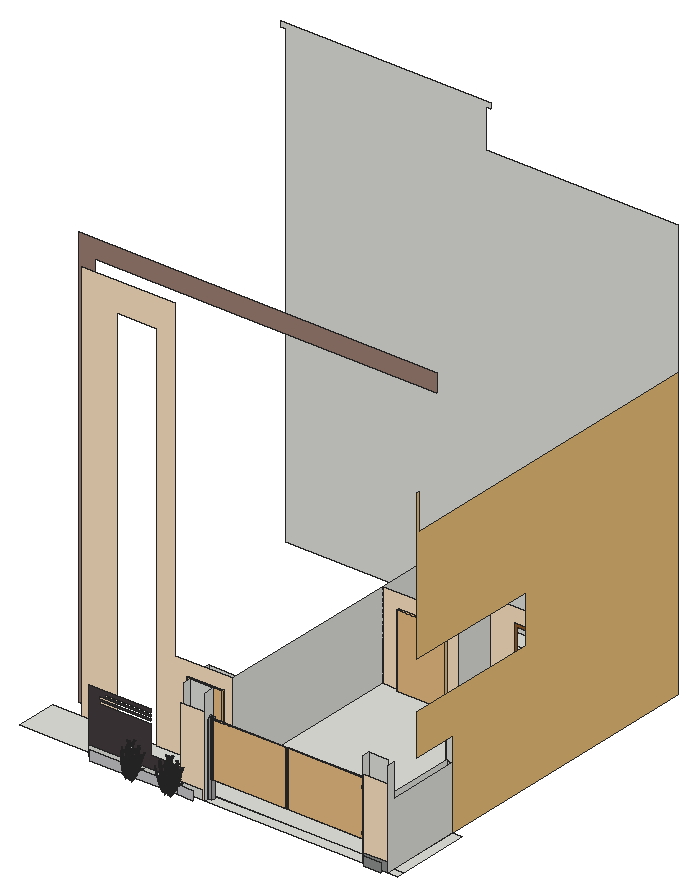
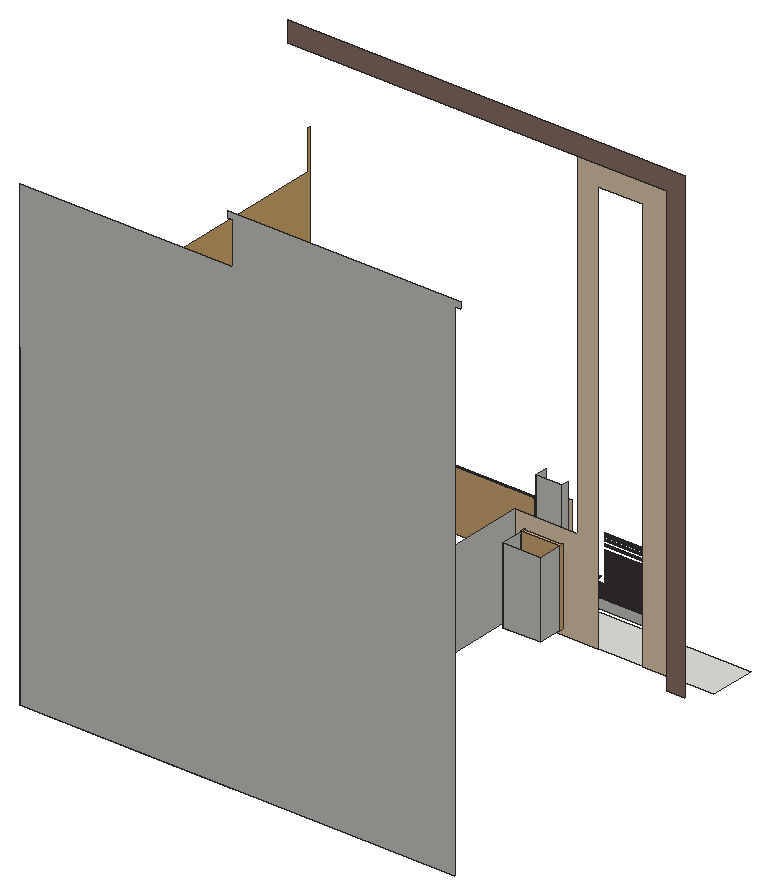
# SketchUp Ruby script. Lengths in inches.
U = 1.inch
M = Sketchup.active_model
def pt(a) = Geom::Point3d.new(a.map { |v| v * U })
def face(e, loops, mat)
  f = e.add_face(loops[0].map { |a| pt(a) })
  loops[1..].each { |l| e.add_face(l.map { |a| pt(a) }).erase! }
  f.material = f.back_material = mat if mat
  f
end
# faces: each face lists its corners as indices into pts; further lists are holes
def faces(e, pts, list, mat = nil) = list.each { |f| face(e, (f[0].is_a?(Array) ? f : [f]).map { |l| l.map { |i| pts[i] } }, mat) }
# xy, xz, yz: faces in a plane at the given z, y or x. An outline is a flat list of corners, or four numbers for a rectangle; further outlines are holes
def ring(l) = l.size == 4 ? [[l[0], l[1]], [l[2], l[1]], [l[2], l[3]], [l[0], l[3]]] : l.each_slice(2).to_a
def flat(e, list, mat, &to3) = list.each { |f| face(e, (f[0].is_a?(Array) ? f : [f]).map { |l| ring(l).map { |u, v| to3.(u, v) } }, mat) }
def xy(e, z, list, mat = nil) = flat(e, list, mat) { |x, y| [x, y, z] }
def xz(e, y, list, mat = nil) = flat(e, list, mat) { |x, z| [x, y, z] }
def yz(e, x, list, mat = nil) = flat(e, list, mat) { |y, z| [x, y, z] }
def lines(e, pts, list) = list.each { |a, b| e.add_line(pt(pts[a]), pt(pts[b])) }
# prism: a flat outline (further loops are holes) pulled along v
def prism(e, loops, v, mat = nil)
  f = face(e, loops, mat); d = Geom::Vector3d.new(v.map { |x| x * U })
  f.pushpull(f.normal.samedirection?(d) ? d.length : -d.length)
end
def box(e, o, s, mat = nil) = prism(e, [[o, [o[0] + s[0], o[1], o[2]], [o[0] + s[0], o[1] + s[1], o[2]], [o[0], o[1] + s[1], o[2]]]], [0, 0, s[2]], mat)
def at(x, y, z, deg = 0) = Geom::Transformation.translation(pt([x, y, z])) * Geom::Transformation.rotation(ORIGIN, Z_AXIS, deg.degrees)
def axes(o, x, y, z) = Geom::Transformation.new([*x, 0, *y, 0, *z, 0, *pt(o).to_a, 1])
def part(name) = M.definitions.add(name)
# library, detail: a bought-in or finely detailed component or shape, given as its bounding box
def library(name, o, s) = part(name).tap { |d| box(d.entities, o, s) }
def detail(e, o, s) = box(e.add_group.entities, o, s)
def put(e, d, t, mat = nil) = e.add_instance(d, t).tap { |i| i.material = mat if mat }
def group(e, t, mat = nil) = e.add_group.tap { |g| g.transformation = t; g.material = mat if mat }.entities
root = M.entities
M.materials.add("Niraj_Skin").color = [158, 128, 115]
M.materials.add("[0012_Bisque]").color = [255, 228, 196]
M.materials.add("[Asphalt New]").color = [67, 60, 62]
M.materials.add("[Blacktop Old 02]").color = [143, 145, 145]
M.materials.add("[Color_003]").color = [170, 170, 170]
M.materials.add("[Metal_Corrogated_Shiny]").color = [193, 193, 193]
M.materials.add("[Polished Concrete New]").color = [200, 200, 203]
M.materials.add("[Wood Floor Parquet]").color = [145, 89, 39]
M.materials.add("[Wood OSB]").color = [240, 195, 122]
M.materials.add("[Wood Veneer 02]").color = [190, 128, 91]
c1 = part("fur_instance\#8")
p = [[-0.25,1.49,0.03],[0.25,-1.49,-0.03],[0.44,-1.47,1.51],[-0.05,1.47,1.57],[0.65,-1.44,3.05],[0.16,1.45,3.11],
  [0.86,-1.42,4.59],[0.38,1.44,4.65],[1.1,-1.39,6.13],[0.62,1.43,6.18],[1.34,-1.35,7.66],[0.875,1.42,7.72],
  [1.6,-1.32,9.19],[1.14,1.41,9.25],[1.88,-1.28,10.72],[1.43,1.41,10.78],[2.18,-1.24,12.25],[1.73,1.41,12.3],
  [2.49,-1.19,13.77],[2.05,1.41,13.82],[2.83,-1.15,15.29],[2.4,1.41,15.34],[3.18,-1.09,16.8],[2.76,1.42,16.85],
  [3.56,-1.03,18.31],[3.14,1.43,18.35],[3.96,-0.97,19.81],[3.55,1.44,19.85],[4.38,-0.91,21.3],[3.99,1.46,21.35],
  [4.84,-0.83,22.78],[4.45,1.48,22.83],[5.32,-0.76,24.26],[4.93,1.51,24.31],[5.82,-0.67,25.73],[5.45,1.54,25.77],
  [6.36,-0.59,27.18],[6,1.57,27.23],[6.93,-0.49,28.625],[6.58,1.61,28.67],[7.54,-0.39,30.05],[7.19,1.66,30.1],
  [8.18,-0.28,31.47],[7.84,1.71,31.51],[8.85,-0.16,32.86],[8.53,1.77,32.9],[9.57,-0.04,34.24],[9.25,1.83,34.27],
  [10.32,0.09,35.59],[10.02,1.9,35.625],[11.12,0.23,36.92],[10.82,1.97,36.95],[11.95,0.38,38.22],[11.67,2.06,38.25],
  [12.84,0.54,39.49],[12.57,2.14,39.52],[13.76,0.71,40.73],[13.51,2.24,40.76],[14.73,0.89,41.93],[14.49,2.34,41.95],
  [15.75,1.08,43.09],[15.52,2.45,43.11],[16.82,1.28,44.2],[16.6,2.5625,44.23],[17.93,1.5,45.27],[17.73,2.68,45.29],
  [19.08,1.73,46.28],[18.9,2.81,46.3],[20.29,1.97,47.24],[20.125,2.93,47.26],[21.53,2.22,48.13],[21.39,3.0625,48.15],
  [22.82,2.5,48.96],[22.7,3.1875,48.98],[24.14,2.8125,49.72],[24.06,3.3,49.73],[25.48,3.27,50.41]]
faces(c1.entities,p,[[0,1,2,3],[3,2,4,5],[5,4,6,7],[7,6,8,9],[9,8,10,11],[11,10,12,13],[13,12,14,15],[15,14,16,17],
  [17,16,18,19],[19,18,20,21],[21,20,22,23],[23,22,24,25],[25,24,26,27],[27,26,28,29],[29,28,30,31],[31,30,32,33],
  [33,32,34,35],[35,34,36,37],[37,36,38,39],[39,38,40,41],[41,40,42,43],[43,42,44,45],[45,44,46,47],[47,46,48,49],
  [49,48,50,51],[51,50,52,53],[53,52,54,55],[55,54,56,57],[57,56,58,59],[59,58,60,61],[61,60,62,63],[63,62,64,65],
  [65,64,66,67],[67,66,68,69],[69,68,70,71],[71,70,72,73],[73,72,74,75],[75,74,76]])
c2 = library("tabla profil",[0,0,0],[95.67,0.85,78.74])
c3 = part("stilp")
box(c3.entities,[0,0,0],[4.72,4.41,106.3])
c4 = part("balama mama")
detail(c4.entities,[0,0,0],[1.18,1.18,2.76])
c5 = part("plastina balamale")
box(c5.entities,[0,0,0],[1.57,0.16,2.76])
c6 = part("balama stilp")
put(c6.entities,c4,at(1.125,0,0))
put(c6.entities,c5,at(0,1.02,0))
c7 = part("Group\#1")
put(c7.entities,c3,at(0,1.18,0))
put(c7.entities,c6,at(3.13,0,92.38))
put(c7.entities,c6,at(3.13,0,33.33))
c8 = library("Group\#2",[0,0,0],[99.09,2.17,78.74])
c9 = part("poarta+metal+2x5m")
g1 = group(c9.entities,at(-0.02,-1.18,-19.69))
put(g1,c2,at(105.29,0.33,27.56),"[Metal_Corrogated_Shiny]")
put(g1,c2,at(6.47,0.33,27.56),"[Metal_Corrogated_Shiny]")
put(g1,c7,at(0,0,0),"[Color_003]")
put(g1,c8,at(4.26,0,27.56),"[Color_003]")
put(g1,c7,axes([207.17,0,0],[-1,0,0],[0,1,0],[0,0,1]),"[Color_003]")
put(g1,c8,axes([202.92,0,27.56],[-1,0,0],[0,1,0],[0,0,1]),"[Color_003]")
c10 = library("curtain (1)",[0,0,0],[91.86,2.24,61.53])
c11 = library("porta+de+madeira",[3.7,-4.82,1.36],[53.55,7.65,83.26])
xy(root,0,[[238.24,86.15,415.52,86.15,415.52,94.44,410.77,94.44,410.77,98.26,238.24,98.26],[415.52,86.15,442.8125,86.15,442.8125,176.35,436.76,176.35,436.76,94.44,415.52,94.44],[442.8125,86.15,453.6875,94.44],[[28.64,90.32,211.95,90.32,211.95,98.26,410.77,98.26,410.77,94.44,436.76,94.44,436.76,176.35,435.86,176.35,435.86,471.23,394.67,471.23,394.67,390.22,313.66,390.22,313.66,346.4375,228.75,346.4375,228.75,136.77,28.64,136.77],[415.79,368,430.67,395.12],[418.11,240,430.67,264.5],[417.11,299.56,430.67,322]],[442.8125,94.44,443,176.35],
  [443,94.44,453.6875,176.35],[435.86,176.35,443,176.35,443,490.875,313.66,490.875,313.66,471.23,435.86,471.23],[418.11,240,430.67,242.37],[418.11,242.37,430.67,264.5],[228.75,346.4375,313.66,471.23],
  [228.75,471.23,313.66,490.875]])
xy(root,5.34,[[181.07,136.77,218.95,164.02]])
xz(root,79.88,[[115.35,0,211.95,10.375],[211.95,0,230.42,10.375]],"[Polished Concrete New]")
xz(root,82.15,[[419.51,0,438.8125,10.375]],"[Blacktop Old 02]")
xz(root,86.15,[[109.08,0,211.95,10.375],[211.95,0,236.6875,10.375]])
xz(root,86.15,[[236.6875,0,238.24,0,238.24,88.875,211.95,88.875,211.95,10.375,236.6875,10.375],[415.52,10.375,442.8125,88.875]],"[0012_Bisque]")
xz(root,86.15,[[109.08,10.375,211.95,10.375,211.95,24.89,178.5,24.89,178.5,55.78,120.75,55.78,120.75,58.72,178.5,58.72,178.5,60.82,120.5,60.82,120.5,63.13,178.5,63.13,178.5,64.89,127.31,64.89,127.31,67.33,178.5,67.33,178.5,70.5625,109.08,70.5625]],"[Asphalt New]")
xz(root,86.15,[[415.52,0,442.8125,10.375]],"[Blacktop Old 02]")
xz(root,94.44,[[415.52,0,436.76,107.1875]])
xz(root,98.26,[[211.95,0,238.24,107.1875]])
xz(root,136.77,[[[60.84,0,99.93,0,99.93,416.99,144.79,416.99,144.79,0,228.75,0,228.75,96.9375,164.91,96.9375,164.91,450.1,60.84,450.1],[181.07,5.34,218.95,81.4]]],"[0012_Bisque]")
xz(root,154.83,[[43.27,0,60.84,0,60.84,450.1,228.75,450.1,228.75,449.78,443,449.78,443,470.41,43.27,470.41]],"Niraj_Skin")
xz(root,164.02,[[181.07,5.34,218.95,81.4]])
xz(root,176.35,[[435.86,0,436.76,0,436.76,70.5625,442.8125,70.5625,442.8125,0,443,0,443,96.9375,435.86,96.9375]])
xz(root,240,[[418.11,0,430.67,78.69]],"[Wood Veneer 02]")
xz(root,264.5,[[418.11,0,418.11,78.69,419.11,78.69,419.11,100.125,430.67,100.125,430.67,0]])
xz(root,299.56,[[417.11,0,430.67,78.27]],"[Wood Veneer 02]")
xz(root,322,[[417.11,0,417.11,78.27,419.11,78.27,419.11,109.68,430.67,109.68,430.67,0]])
xz(root,346.4375,[[247.19,0,293.21,81.21]])
xz(root,346.4375,[[228.75,0,247.19,0,247.19,81.21,293.21,81.21,293.21,0,313.66,0,313.66,96.9375,228.75,96.9375]],"[0012_Bisque]")
xz(root,368,[[415.79,0,430.67,78.27]],"[Wood Veneer 02]")
xz(root,390.22,[[[313.66,0,394.67,96.9375],[341.37,19.24,374.18,80.3]]],"[0012_Bisque]")
xz(root,390.22,[[[341.37,19.24,374.18,80.3],[343.67,21.55,371.875,78]]],"[Wood Floor Parquet]")
xz(root,395.12,[[415.79,0,415.79,78.27,419.11,78.27,419.11,109.68,430.67,109.68,430.67,0]])
xz(root,471.23,[[394.67,0,435.86,96.9375]],"[0012_Bisque]")
xz(root,490.875,[[5.25,0,5.25,513.13,0,513.13,0,519.625,233.81,519.625,233.81,513.13,228.75,513.13,228.75,470.41,443,470.41,443,0]])
yz(root,181.07,[[136.77,5.34,164.02,81.4]])
yz(root,211.95,[[90.32,0,98.26,107.1875]])
yz(root,218.95,[[136.77,5.34,164.02,81.4]])
yz(root,228.75,[[136.77,0,346.4375,96.9375],[346.4375,0,471.23,96.9375]])
yz(root,238.24,[[86.15,0,98.26,107.1875]])
yz(root,313.66,[[346.4375,0,390.22,96.9375]])
yz(root,394.67,[[390.22,0,471.23,96.9375]])
yz(root,415.52,[[86.15,0,94.44,107.1875]])
yz(root,415.79,[[368,0,395.12,78.27]],"[Wood Veneer 02]")
yz(root,417.11,[[299.56,0,322,78.27]],"[Wood Veneer 02]")
yz(root,418.11,[[240,0,264.5,78.69]],"[Wood Veneer 02]")
yz(root,430.67,[[240,0,242.37,0,242.37,78.73,242.25,78.69,240,78.69],[242.37,0,264.5,0,264.5,84.8125,242.37,78.73],[299.56,0,322,0,322,80.77,302,78.27,299.56,78.27],[368,0,395.12,0,395.12,109.68,372.37,109.68,372.37,78.27,368,78.27]])
yz(root,435.86,[[176.35,0,471.23,96.9375]])
yz(root,436.76,[[94.44,0,176.35,70.5625]])
yz(root,442.8125,[[86.15,0,176.35,0,176.35,70.5625,94.44,70.5625,94.44,107.1875,86.15,107.1875]])
yz(root,443,[[176.35,0,490.875,0,490.875,322.1875,129.24,322.1875,129.24,361.9375,126.77,361.9375,126.77,195.98,278.53,195.98,278.53,142.87,126.77,142.87,126.77,96.9375,176.35,96.9375]],"[Wood OSB]")
p = [[313.66,471.23,0],[313.66,471.23,96.9375],[229.47,346.4375,0],[229.47,176.35,0]]
lines(root,p,[[0,1],[2,3]])
put(root,c1,axes([206.91,69.77,2.21],[0.10395,0.11836,-0.12851],[-0.11439,0.07411,-0.26217],[-0.07351,0.08501,0.2481]))
put(root,c1,axes([201.6,71.41,5.67],[-0.08139,0.23064,-0.15312],[-0.1699,-0.05496,-0.32193],[-0.16391,-0.02606,0.43057]))
put(root,c1,axes([162.83,72.15,2.37],[0.12897,-0.08882,0.30598],[0.12311,0.13439,-0.14076],[-0.0848,0.09806,0.28618]))
put(root,c1,axes([206.14,72.15,2.37],[0.12897,-0.08882,0.30598],[0.12311,0.13439,-0.14076],[-0.0848,0.09806,0.28618]))
put(root,c1,axes([169.21,72.82,2.47],[-0.12598,-0.09298,0.35138],[0.14548,-0.16001,0.09177],[0.09178,0.08501,0.30971]))
put(root,c1,axes([212.52,72.82,2.47],[-0.12598,-0.09298,0.35138],[0.14548,-0.16001,0.09177],[0.09178,0.08501,0.30971]))
put(root,c1,axes([168.61,74.05,5.45],[0.17475,-0.1628,0.03799],[0.13362,0.1403,-0.32315],[0.08136,0.06328,0.41208]))
put(root,c1,axes([211.92,74.05,5.45],[0.17475,-0.1628,0.03799],[0.13362,0.1403,-0.32315],[0.08136,0.06328,0.41208]))
put(root,c1,axes([167.55,73.21,2.36],[-0.04728,-0.14736,0.35137],[0.1919,-0.08682,-0.02284],[0.06183,0.09936,0.30152]))
put(root,c1,axes([210.87,73.21,2.36],[-0.04728,-0.14736,0.35137],[0.1919,-0.08682,-0.02284],[0.06183,0.09936,0.30152]))
put(root,c1,axes([168.81,74.19,4.9],[-0.12567,-0.14648,0.32324],[0.17955,-0.15616,0.02426],[0.08105,0.06304,0.41053]))
put(root,c1,axes([212.12,74.19,4.9],[-0.12567,-0.14648,0.32324],[0.17955,-0.15616,0.02426],[0.08105,0.06304,0.41053]))
put(root,c1,axes([169.69,70.52,3.26],[-0.05675,0.18901,-0.12396],[-0.14509,-0.01855,0.32364],[0.12915,0.03597,0.29172]))
put(root,c1,axes([213,70.52,3.26],[-0.05675,0.18901,-0.12396],[-0.14509,-0.01855,0.32364],[0.12915,0.03597,0.29172]))
put(root,c1,axes([162.25,73.15,3.23],[0.03058,-0.16302,0.35291],[0.18885,0.05742,0.07777],[-0.09099,0.10522,0.30707]))
put(root,c1,axes([205.5625,73.15,3.23],[0.03058,-0.16302,0.35291],[0.18885,0.05742,0.07777],[-0.09099,0.10522,0.30707]))
put(root,c1,axes([166.74,72.07,10.54],[-0.19584,0.16179,-0.00169],[-0.1515,-0.17581,0.15196],[0.03573,-0.00363,0.539]))
put(root,c1,axes([210.06,72.07,10.54],[-0.19584,0.16179,-0.00169],[-0.1515,-0.17581,0.15196],[0.03573,-0.00363,0.539]))
put(root,c1,axes([162.77,70.35,2.66],[0.12204,0.11956,-0.03437],[-0.09323,0.10261,-0.31254],[-0.10097,0.07745,0.26536]))
put(root,c1,axes([206.08,70.35,2.66],[0.12204,0.11956,-0.03437],[-0.09323,0.10261,-0.31254],[-0.10097,0.07745,0.26536]))
put(root,c1,axes([166.49,71.18,8.18],[0.03623,0.20627,-0.12936],[-0.21911,0.05324,0.03667],[0.02079,0.00357,0.48088]))
put(root,c1,axes([209.8,71.18,8.18],[0.03623,0.20627,-0.12936],[-0.21911,0.05324,0.03667],[0.02079,0.00357,0.48088]))
put(root,c1,axes([162.41,72.88,7.12],[0.2158,0.0049,0.14651],[-0.01279,0.21776,-0.18636],[-0.08047,0.03325,0.45875]))
put(root,c1,axes([205.72,72.88,7.12],[0.2158,0.0049,0.14651],[-0.01279,0.21776,-0.18636],[-0.08047,0.03325,0.45875]))
put(root,c1,axes([164.05,70.84,3.85],[-0.12886,0.11444,-0.22997],[-0.12949,-0.11784,0.12414],[-0.04678,0.07389,0.33152]))
put(root,c1,axes([207.36,70.84,3.85],[-0.12886,0.11444,-0.22997],[-0.12949,-0.11784,0.12414],[-0.04678,0.07389,0.33152]))
put(root,c1,axes([165.51,71.02,2.9375],[0.17646,0.02205,-0.09309],[-0.04854,0.13883,-0.29657],[0.00073,0.10392,0.26687]))
put(root,c1,axes([208.82,71.02,2.9375],[0.17646,0.02205,-0.09309],[-0.04854,0.13883,-0.29657],[0.00073,0.10392,0.26687]))
put(root,c1,axes([165.39,72.23,11.89],[0.11288,0.21144,-0.04258],[-0.23471,0.1258,-0.00774],[-0.00125,-0.03681,0.58142]))
put(root,c1,axes([208.7,72.23,11.89],[0.11288,0.21144,-0.04258],[-0.23471,0.1258,-0.00774],[-0.00125,-0.03681,0.58142]))
put(root,c1,axes([159.4,71.5,4.78],[0.05993,0.19956,0.02934],[-0.16765,0.09615,-0.32784],[-0.14862,0.00196,0.40149]))
put(root,c1,axes([202.71,71.5,4.78],[0.05993,0.19956,0.02934],[-0.16765,0.09615,-0.32784],[-0.14862,0.00196,0.40149]))
put(root,c1,axes([164.65,71.8,9.23],[-0.15948,0.17543,-0.11844],[-0.17074,-0.13846,0.07646],[-0.0175,0.01182,0.50519]))
put(root,c1,axes([207.96,71.8,9.23],[-0.15948,0.17543,-0.11844],[-0.17074,-0.13846,0.07646],[-0.0175,0.01182,0.50519]))
put(root,c1,axes([169.24,70.62,2.31],[-0.02741,0.17392,-0.23076],[-0.16029,0.02766,0.23757],[0.10574,0.05755,0.28081]))
put(root,c1,axes([212.55,70.62,2.31],[-0.02741,0.17392,-0.23076],[-0.16029,0.02766,0.23757],[0.10574,0.05755,0.28081]))
put(root,c1,axes([165.59,73.07,10.61],[-0.22966,0.11975,-0.02971],[-0.1055,-0.20961,0.14888],[0.00986,0.00949,0.54546]))
put(root,c1,axes([208.9,73.07,10.61],[-0.22966,0.11975,-0.02971],[-0.1055,-0.20961,0.14888],[0.00986,0.00949,0.54546]))
put(root,c1,axes([161.59,71.875,4.67],[0.149,0.11824,0.07488],[-0.1012,0.16059,-0.29075],[-0.11547,0.04466,0.37315]))
put(root,c1,axes([204.9,71.875,4.67],[0.149,0.11824,0.07488],[-0.1012,0.16059,-0.29075],[-0.11547,0.04466,0.37315]))
put(root,c1,axes([203.16,71.44,3.41],[-0.06018,0.17755,-0.31983],[-0.13865,-0.10086,-0.20049],[-0.15862,0.04585,0.31318]))
put(root,c1,axes([202.73,72.31,7.63],[-0.04995,0.23864,-0.11124],[-0.21419,-0.02204,-0.24055],[-0.12191,-0.01612,0.49664]))
put(root,c1,axes([161.89,71.77,3.15],[-0.12441,0.08913,-0.33358],[-0.11522,-0.1494,0.09624],[-0.1115,0.08552,0.29301]))
put(root,c1,axes([205.21,71.77,3.15],[-0.12441,0.08913,-0.33358],[-0.11522,-0.1494,0.09624],[-0.1115,0.08552,0.29301]))
put(root,c1,axes([169.99,72.21,7.55],[0.06433,0.21786,-0.19116],[-0.21809,0.08663,0.16557],[0.09246,-0.00116,0.48782]))
put(root,c1,axes([213.3,72.21,7.55],[0.06433,0.21786,-0.19116],[-0.21809,0.08663,0.16557],[0.09246,-0.00116,0.48782]))
put(root,c1,axes([169.59,73.11,3.22],[-0.18323,0.03397,0.2678],[0.02904,-0.19802,0.26654],[0.12063,0.06566,0.32036]))
put(root,c1,axes([212.9,73.11,3.22],[-0.18323,0.03397,0.2678],[0.02904,-0.19802,0.26654],[0.12063,0.06566,0.32036]))
put(root,c1,axes([164.06,71.89,5.04],[-0.16185,0.10098,-0.22361],[-0.11509,-0.14728,0.17524],[-0.05085,0.08033,0.3604]))
put(root,c1,axes([207.37,71.89,5.04],[-0.16185,0.10098,-0.22361],[-0.11509,-0.14728,0.17524],[-0.05085,0.08033,0.3604]))
put(root,c1,axes([166.31,71.96,6.02],[-0.1319,0.16634,-0.13442],[-0.16484,-0.10583,0.16664],[0.0172,0.04548,0.42308]))
put(root,c1,axes([209.62,71.96,6.02],[-0.1319,0.16634,-0.13442],[-0.16484,-0.10583,0.16664],[0.0172,0.04548,0.42308]))
put(root,c1,axes([166.24,72.08,3.71],[0.16157,0.07757,-0.19831],[-0.11325,0.15562,-0.18994],[0.0239,0.07619,0.35007]))
put(root,c1,axes([209.55,72.08,3.71],[0.16157,0.07757,-0.19831],[-0.11325,0.15562,-0.18994],[0.0239,0.07619,0.35007]))
put(root,c1,axes([164.1,72.54,4.23],[-0.18808,0.05687,-0.16759],[-0.06647,-0.17012,0.23097],[-0.05108,0.08069,0.36201]))
put(root,c1,axes([207.41,72.54,4.23],[-0.18808,0.05687,-0.16759],[-0.06647,-0.17012,0.23097],[-0.05108,0.08069,0.36201]))
put(root,c1,axes([165.86,71.66,2.72],[-0.17438,0.07052,-0.11324],[-0.07295,-0.12692,0.30042],[0.00076,0.10733,0.27565]))
put(root,c1,axes([209.17,71.66,2.72],[-0.17438,0.07052,-0.11324],[-0.07295,-0.12692,0.30042],[0.00076,0.10733,0.27565]))
put(root,c1,axes([159.29,73.21,2.46],[0.15352,0.06911,0.26676],[-0.03494,0.20117,-0.28887],[-0.16523,0.04776,0.32623]))
put(root,c1,axes([202.6,73.21,2.46],[0.15352,0.06911,0.26676],[-0.03494,0.20117,-0.28887],[-0.16523,0.04776,0.32623]))
put(root,c1,axes([165.14,73.51,5.21],[-0.21697,-0.00618,0.04885],[0.02773,-0.18874,0.29817],[-0.00075,0.0894,0.38532]))
put(root,c1,axes([208.45,73.51,5.21],[-0.21697,-0.00618,0.04885],[0.02773,-0.18874,0.29817],[-0.00075,0.0894,0.38532]))
put(root,c1,axes([167.67,72.27,8.23],[0.08086,0.19655,-0.23287],[-0.213,0.10459,0.05528],[0.05877,0.03065,0.4692]))
put(root,c1,axes([210.99,72.27,8.23],[0.08086,0.19655,-0.23287],[-0.213,0.10459,0.05528],[0.05877,0.03065,0.4692]))
put(root,c1,axes([160.4,72.72,7.94],[-0.0789,0.22714,-0.18379],[-0.20548,-0.06456,-0.18143],[-0.11262,0.00359,0.48952]))
put(root,c1,axes([203.71,72.72,7.94],[-0.0789,0.22714,-0.18379],[-0.20548,-0.06456,-0.18143],[-0.11262,0.00359,0.48952]))
put(root,c1,axes([166.54,74.67,4.57],[-0.18748,-0.08453,0.22152],[0.12512,-0.17975,0.22209],[0.0273,0.08703,0.39989]))
put(root,c1,axes([209.85,74.67,4.57],[-0.18748,-0.08453,0.22152],[0.12512,-0.17975,0.22209],[0.0273,0.08703,0.39989]))
put(root,c1,axes([167.96,71.4,2.67],[0.02265,0.14627,-0.32338],[-0.18321,0.06424,0.06],[0.05776,0.09281,0.28164]))
put(root,c1,axes([211.28,71.4,2.67],[0.02265,0.14627,-0.32338],[-0.18321,0.06424,0.06],[0.05776,0.09281,0.28164]))
put(root,c1,axes([168.93,72.78,9.83],[-0.06671,0.24175,-0.07521],[-0.22931,-0.04686,0.25475],[0.09711,-0.00122,0.51237]))
put(root,c1,axes([212.24,72.78,9.83],[-0.06671,0.24175,-0.07521],[-0.22931,-0.04686,0.25475],[0.09711,-0.00122,0.51237]))
put(root,c1,axes([163.52,72.73,10.38],[-0.03892,0.23857,-0.13916],[-0.24331,-0.01786,-0.06409],[-0.04532,0.0056,0.5395]))
put(root,c1,axes([206.83,72.73,10.38],[-0.03892,0.23857,-0.13916],[-0.24331,-0.01786,-0.06409],[-0.04532,0.0056,0.5395]))
put(root,c1,axes([164.64,72.03,5.51],[0.14274,0.1248,-0.18106],[-0.14873,0.12853,-0.2232],[-0.02656,0.08555,0.36591]))
put(root,c1,axes([207.96,72.03,5.51],[0.14274,0.1248,-0.18106],[-0.14873,0.12853,-0.2232],[-0.02656,0.08555,0.36591]))
put(root,c1,axes([163.76,72.71,6.8],[0.14854,0.14611,-0.10639],[-0.16099,0.14725,-0.20019],[-0.04301,0.04934,0.44533]))
put(root,c1,axes([207.07,72.71,6.8],[0.14854,0.14611,-0.10639],[-0.16099,0.14725,-0.20019],[-0.04301,0.04934,0.44533]))
put(root,c1,axes([161.33,74.08,7.08],[0.21224,0.07306,0.08848],[-0.08036,0.21667,-0.23259],[-0.08448,0.0349,0.48158]))
put(root,c1,axes([204.64,74.08,7.08],[0.21224,0.07306,0.08848],[-0.08036,0.21667,-0.23259],[-0.08448,0.0349,0.48158]))
put(root,c1,axes([161.38,73.15,2.17],[-0.14657,0.06865,-0.32949],[-0.09952,-0.16829,0.15169],[-0.11649,0.08935,0.30613]))
put(root,c1,axes([204.7,73.15,2.17],[-0.14657,0.06865,-0.32949],[-0.09952,-0.16829,0.15169],[-0.11649,0.08935,0.30613]))
put(root,c1,axes([163.86,73.3,9.57],[0.10044,0.20522,-0.10286],[-0.22219,0.11383,-0.10772],[-0.03192,0.01018,0.52996]))
put(root,c1,axes([207.18,73.3,9.57],[0.10044,0.20522,-0.10286],[-0.22219,0.11383,-0.10772],[-0.03192,0.01018,0.52996]))
put(root,c1,axes([164.01,73.95,11.01],[0.19334,0.14897,-0.05271],[-0.17118,0.19893,-0.14866],[-0.0338,0.01079,0.56126]))
put(root,c1,axes([207.33,73.95,11.01],[0.19334,0.14897,-0.05271],[-0.17118,0.19893,-0.14866],[-0.0338,0.01079,0.56126]))
put(root,c1,axes([169.15,73.23,7.55],[-0.1067,0.21804,-0.07354],[-0.20586,-0.08261,0.23931],[0.07827,0.01663,0.48727]))
put(root,c1,axes([212.46,73.23,7.55],[-0.1067,0.21804,-0.07354],[-0.20586,-0.08261,0.23931],[0.07827,0.01663,0.48727]))
put(root,c1,axes([160.73,72.97,5.79],[-0.09952,0.18231,-0.31022],[-0.16857,-0.11721,-0.10121],[-0.1255,0.04853,0.40556]))
put(root,c1,axes([204.04,72.97,5.79],[-0.09952,0.18231,-0.31022],[-0.16857,-0.11721,-0.10121],[-0.1255,0.04853,0.40556]))
put(root,c1,axes([166.15,73.26,2.17],[0.19789,0.01674,-0.08664],[-0.04397,0.1548,-0.33323],[0.00081,0.11511,0.29561]))
put(root,c1,axes([209.47,73.26,2.17],[0.19789,0.01674,-0.08664],[-0.04397,0.1548,-0.33323],[0.00081,0.11511,0.29561]))
put(root,c1,axes([167.9375,73.73,3.08],[0.19779,0.00085,-0.20861],[-0.06023,0.17892,-0.30359],[0.06469,0.10395,0.31543]))
put(root,c1,axes([211.25,73.73,3.08],[0.19779,0.00085,-0.20861],[-0.06023,0.17892,-0.30359],[0.06469,0.10395,0.31543]))
put(root,c1,axes([163.03,73.32,2.28],[-0.17971,0.05049,-0.21333],[-0.08082,-0.15328,0.27859],[-0.06056,0.11282,0.29972]))
put(root,c1,axes([206.34,73.32,2.28],[-0.17971,0.05049,-0.21333],[-0.08082,-0.15328,0.27859],[-0.06056,0.11282,0.29972]))
put(root,c1,axes([168.21,73.24,9.34],[-0.0236,0.24008,-0.16159],[-0.23761,0.00409,0.20091],[0.0806,0.01712,0.5018]))
put(root,c1,axes([211.53,73.24,9.34],[-0.0236,0.24008,-0.16159],[-0.23761,0.00409,0.20091],[0.0806,0.01712,0.5018]))
put(root,c1,axes([163.99,73.01,8.11],[-0.03105,0.21618,-0.23248],[-0.22713,-0.0199,-0.04743],[-0.04502,0.05164,0.46606]))
put(root,c1,axes([207.31,73.01,8.11],[-0.03105,0.21618,-0.23248],[-0.22713,-0.0199,-0.04743],[-0.04502,0.05164,0.46606]))
put(root,c1,axes([165.98,73.29,3.75],[-0.13558,0.14856,-0.21429],[-0.16001,-0.10351,0.19496],[-0.00072,0.08572,0.36945]))
put(root,c1,axes([209.29,73.29,3.75],[-0.13558,0.14856,-0.21429],[-0.16001,-0.10351,0.19496],[-0.00072,0.08572,0.36945]))
put(root,c1,axes([162.81,74.14,8.77],[-0.1589,0.17803,-0.2479],[-0.17756,-0.14881,0.0508],[-0.06832,0.04712,0.49383]))
put(root,c1,axes([206.12,74.14,8.77],[-0.1589,0.17803,-0.2479],[-0.17756,-0.14881,0.0508],[-0.06832,0.04712,0.49383]))
put(root,c1,axes([163.4375,73.78,3.31],[0.1975,0.05806,-0.0072],[-0.05058,0.15655,-0.36297],[-0.06266,0.11673,0.31011]))
put(root,c1,axes([206.75,73.78,3.31],[0.1975,0.05806,-0.0072],[-0.05058,0.15655,-0.36297],[-0.06266,0.11673,0.31011]))
put(root,c1,axes([161.34,75.29,3.79],[0.19488,-0.04118,0.27862],[0.0814,0.18631,-0.28554],[-0.10045,0.11615,0.33899]))
put(root,c1,axes([204.65,75.29,3.79],[0.19488,-0.04118,0.27862],[0.0814,0.18631,-0.28554],[-0.10045,0.11615,0.33899]))
put(root,c1,axes([163.5,73.25,2.8],[-0.05838,0.1486,-0.35065],[-0.18856,-0.06365,0.02437],[-0.06066,0.11302,0.30025]))
put(root,c1,axes([206.81,73.25,2.8],[-0.05838,0.1486,-0.35065],[-0.18856,-0.06365,0.02437],[-0.06066,0.11302,0.30025]))
put(root,c1,axes([170.92,74.49,6.625],[-0.08095,0.24089,-0.09572],[-0.20653,-0.05261,0.34972],[0.13417,0.02289,0.45313]))
put(root,c1,axes([214.24,74.49,6.625],[-0.08095,0.24089,-0.09572],[-0.20653,-0.05261,0.34972],[0.13417,0.02289,0.45313]))
put(root,c1,axes([163.34,78.21,5.26],[0.05792,-0.21665,0.35228],[0.2474,0.04272,-0.03732],[-0.03274,0.10545,0.45101]))
put(root,c1,axes([206.65,78.21,5.26],[0.05792,-0.21665,0.35228],[0.2474,0.04272,-0.03732],[-0.03274,0.10545,0.45101]))
put(root,c1,axes([165.86,77.59,4.875],[0.18259,-0.1619,0.22728],[0.17109,0.14301,-0.26039],[-0.00086,0.10227,0.44077]))
put(root,c1,axes([209.17,77.59,4.875],[0.18259,-0.1619,0.22728],[0.17109,0.14301,-0.26039],[-0.00086,0.10227,0.44077]))
put(root,c1,axes([162.54,74.33,7.22],[0.04781,0.21803,-0.18144],[-0.22564,0.05394,-0.16456],[-0.06613,0.04562,0.47803]))
put(root,c1,axes([205.85,74.33,7.22],[0.04781,0.21803,-0.18144],[-0.22564,0.05394,-0.16456],[-0.06613,0.04562,0.47803]))
put(root,c1,axes([169.51,76.41,4.89],[-0.23752,0.04727,0.17981],[0.00037,-0.22718,0.3018],[0.08784,0.06833,0.44492]))
put(root,c1,axes([212.82,76.41,4.89],[-0.23752,0.04727,0.17981],[0.00037,-0.22718,0.3018],[0.08784,0.06833,0.44492]))
put(root,c1,axes([161.33,75.91,4.37],[0.22314,0.03503,0.11397],[-0.0252,0.21097,-0.3146],[-0.08653,0.08429,0.4222]))
put(root,c1,axes([204.64,75.91,4.37],[0.22314,0.03503,0.11397],[-0.0252,0.21097,-0.3146],[-0.08653,0.08429,0.4222]))
put(root,c1,axes([164.27,77.82,5.35],[-0.20442,-0.12057,0.16665],[0.14603,-0.18202,0.30806],[-0.03237,0.10426,0.44592]))
put(root,c1,axes([207.59,77.82,5.35],[-0.20442,-0.12057,0.16665],[0.14603,-0.18202,0.30806],[-0.03237,0.10426,0.44592]))
put(root,c1,axes([166.8125,74.13,3.53],[-0.15443,0.14355,-0.21021],[-0.15015,-0.09516,0.30489],[0.0337,0.11705,0.31784]))
put(root,c1,axes([210.125,74.13,3.53],[-0.15443,0.14355,-0.21021],[-0.15015,-0.09516,0.30489],[0.0337,0.11705,0.31784]))
put(root,c1,axes([164.45,74.42,2.61],[-0.08555,0.15021,-0.34626],[-0.19424,-0.0665,0.11459],[-0.03163,0.1226,0.31264]))
put(root,c1,axes([207.77,74.42,2.61],[-0.08555,0.15021,-0.34626],[-0.19424,-0.0665,0.11459],[-0.03163,0.1226,0.31264]))
put(root,c1,axes([162.17,76.73,7.24],[-0.18658,0.14503,-0.30144],[-0.1645,-0.17028,0.18908],[-0.06369,0.10062,0.4514]))
put(root,c1,axes([205.49,76.73,7.24],[-0.18658,0.14503,-0.30144],[-0.1645,-0.17028,0.18908],[-0.06369,0.10062,0.4514]))
put(root,c1,axes([166.66,77.37,4.57],[-0.22222,0.12257,-0.08636],[-0.10729,-0.17964,0.33239],[0.02989,0.09528,0.43781]))
put(root,c1,axes([209.98,77.37,4.57],[-0.22222,0.12257,-0.08636],[-0.10729,-0.17964,0.33239],[0.02989,0.09528,0.43781]))
put(root,c1,axes([165.86,76.54,7.21],[0.16049,0.15534,-0.27829],[-0.19592,0.15388,-0.21201],[-0.00087,0.10351,0.44615]))
put(root,c1,axes([209.17,76.54,7.21],[0.16049,0.15534,-0.27829],[-0.19592,0.15388,-0.21201],[-0.00087,0.10351,0.44615]))
put(root,c1,axes([167.04,78.43,4.74],[-0.24957,0.08322,-0.01695],[-0.05226,-0.18613,0.43808],[0.0399,0.13857,0.37627]))
put(root,c1,axes([210.36,78.43,4.74],[-0.24957,0.08322,-0.01695],[-0.05226,-0.18613,0.43808],[0.0399,0.13857,0.37627]))
put(root,c9,axes([238.26,91.36,15.14],[0.8536,0,0],[0,0.76901,0],[0,0,0.76901]))
put(root,c10,axes([180.11,134.51,5.34],[0.42277,0,0],[0,2.7574,0],[0,0,1.24538]))
put(root,c11,at(243.49,348.48,-3.32))
